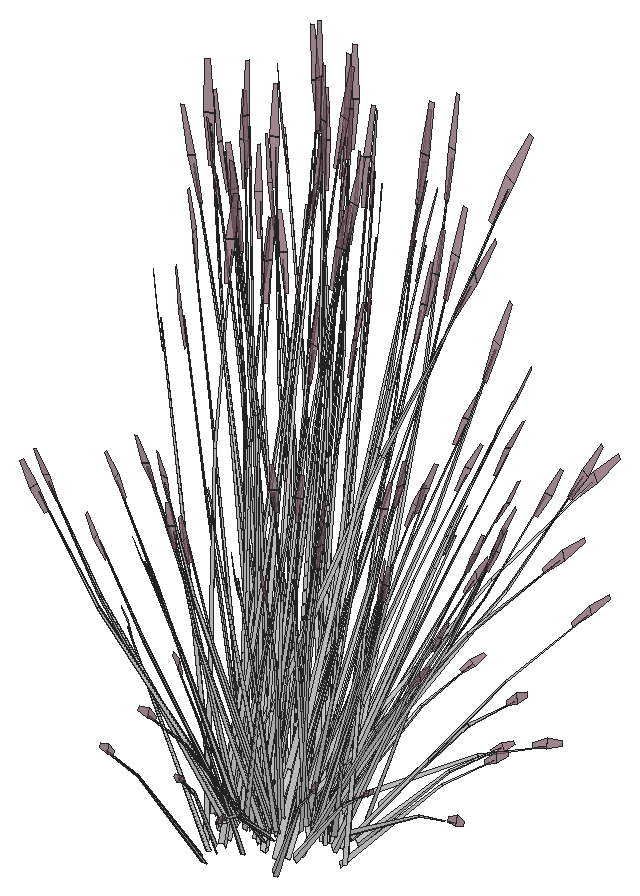
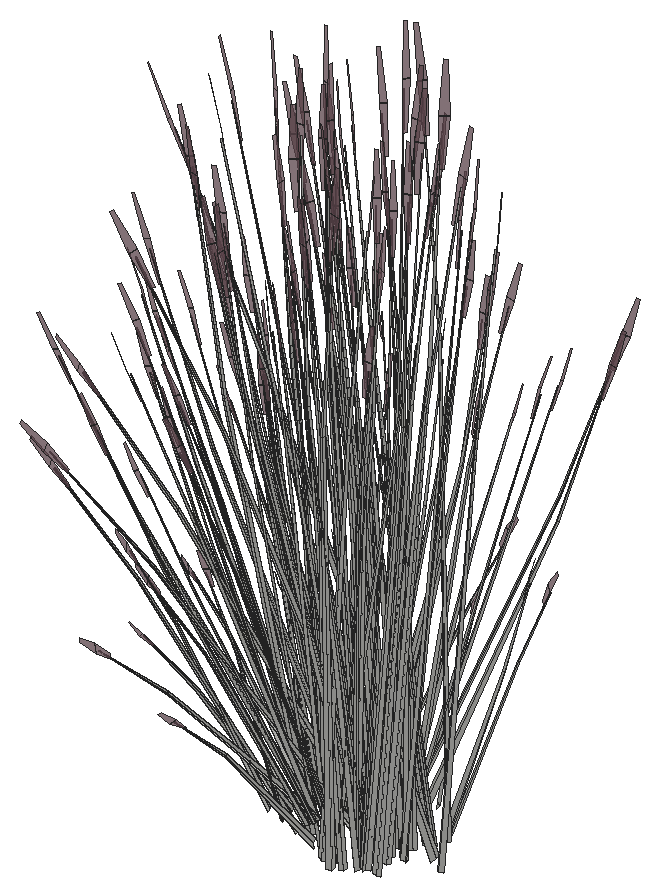
# SketchUp Ruby script. Lengths in inches.
U = 1.inch
M = Sketchup.active_model
def pt(a) = Geom::Point3d.new(a.map { |v| v * U })
def face(e, loops, mat)
  f = e.add_face(loops[0].map { |a| pt(a) })
  loops[1..].each { |l| e.add_face(l.map { |a| pt(a) }).erase! }
  f.material = f.back_material = mat if mat
  f
end
# faces: each face lists its corners as indices into pts; further lists are holes
def faces(e, pts, list, mat = nil) = list.each { |f| face(e, (f[0].is_a?(Array) ? f : [f]).map { |l| l.map { |i| pts[i] } }, mat) }
# xy, xz, yz: faces in a plane at the given z, y or x. An outline is a flat list of corners, or four numbers for a rectangle; further outlines are holes
def ring(l) = l.size == 4 ? [[l[0], l[1]], [l[2], l[1]], [l[2], l[3]], [l[0], l[3]]] : l.each_slice(2).to_a
def flat(e, list, mat, &to3) = list.each { |f| face(e, (f[0].is_a?(Array) ? f : [f]).map { |l| ring(l).map { |u, v| to3.(u, v) } }, mat) }
def xy(e, z, list, mat = nil) = flat(e, list, mat) { |x, y| [x, y, z] }
def xz(e, y, list, mat = nil) = flat(e, list, mat) { |x, z| [x, y, z] }
def yz(e, x, list, mat = nil) = flat(e, list, mat) { |y, z| [x, y, z] }
def lines(e, pts, list) = list.each { |a, b| e.add_line(pt(pts[a]), pt(pts[b])) }
# prism: a flat outline (further loops are holes) pulled along v
def prism(e, loops, v, mat = nil)
  f = face(e, loops, mat); d = Geom::Vector3d.new(v.map { |x| x * U })
  f.pushpull(f.normal.samedirection?(d) ? d.length : -d.length)
end
def box(e, o, s, mat = nil) = prism(e, [[o, [o[0] + s[0], o[1], o[2]], [o[0] + s[0], o[1] + s[1], o[2]], [o[0], o[1] + s[1], o[2]]]], [0, 0, s[2]], mat)
def at(x, y, z, deg = 0) = Geom::Transformation.translation(pt([x, y, z])) * Geom::Transformation.rotation(ORIGIN, Z_AXIS, deg.degrees)
def axes(o, x, y, z) = Geom::Transformation.new([*x, 0, *y, 0, *z, 0, *pt(o).to_a, 1])
def part(name) = M.definitions.add(name)
# library, detail: a bought-in or finely detailed component or shape, given as its bounding box
def library(name, o, s) = part(name).tap { |d| box(d.entities, o, s) }
def detail(e, o, s) = box(e.add_group.entities, o, s)
def put(e, d, t, mat = nil) = e.add_instance(d, t).tap { |i| i.material = mat if mat }
def group(e, t, mat = nil) = e.add_group.tap { |g| g.transformation = t; g.material = mat if mat }.entities
root = M.entities
M.materials.add("LightPink_Translucent").color = [144, 107, 117]
M.materials["LightPink_Translucent"].alpha = 0.75
c1 = part("blade")
p = [[2.15,0.21,22],[0,0.17,0],[0.09,0.45,0],[2.18,0.31,22],[2.29,0.31,22],[0.38,0.45,0],
  [2.48,0.24,33],[2.49,0.24,33],[2.48,0.22,33]]
faces(c1.entities,p,[[0,1,2,3],[4,5,2,3],[6,3,4,7],[8,0,3,6]])
c2 = part("seeds")
p = [[0.3,-0.1,1.38],[-0.01,-0.03,1.59],[-0.01,-0.03,0.03],[0.14,-0.07,-0.07],[0.29,-0.03,3],[0.15,0.01,3.11]]
faces(c2.entities,p,[[0,1,2,3],[1,0,4,5]],"LightPink_Translucent")
c3 = part("blade with seeds")
put(c3.entities,c1,at(0,0,0))
put(c3.entities,c2,axes([2.4,0.25,30.99],[1.5799,-0.05474,1.17369],[-0.12525,1.92788,0.29478],[-0.07173,-0.02425,1.56792]))
put(root,c3,axes([266.18,258.16,16.92],[-1.20468,-0.25962,-0.51099],[0.41292,-0.89013,-0.3958],[-0.11046,-0.35838,0.97773]))
put(root,c3,axes([261.53,261.37,14.26],[0.85545,-0.64616,-0.30978],[0.85545,0.64616,0.30978],[0,-0.20813,1.38974]))
put(root,c3,axes([265.39,257.19,14.36],[-0.84686,0.59414,-0.03893],[-0.77596,-0.65071,-0.17649],[-0.05463,-0.18438,0.58215]))
put(root,c3,axes([265.05,263.05,14.6],[1.54892,0.2182,0.45755],[-0.31522,1.23236,0.17955],[-0.22636,-0.119,1.58856]))
put(root,c3,axes([264.65,262.83,14.95],[-0.59459,0.93321,0.44739],[-1.23546,-0.44912,-0.21531],[0,-0.21512,1.43643]))
put(root,c3,axes([266.61,258.33,17.22],[-0.5849,-0.8421,-0.71045],[1.20401,-0.4693,0.08574],[-0.13677,-0.40688,1.00501]))
put(root,c3,axes([264.22,265.02,14.71],[1.31687,-0.27488,0.17642],[0.32517,1.02297,0.35086],[-0.11745,-0.14905,1.60407]))
put(root,c3,axes([265.92,265.18,14.43],[-1.23546,-0.46496,0],[0.59459,-0.96613,0],[0,0,1.62707]))
put(root,c3,axes([266.84,258.46,17.29],[-0.36946,0.79643,0.35414],[-1.07787,-0.23229,-0.4572],[-0.09883,-0.32066,0.87481]))
put(root,c3,axes([268.14,265.08,14.71],[0.35402,-1.02926,0.17642],[1.29548,0.29127,0.35086],[-0.22379,0.00501,1.60407]))
put(root,c3,axes([267.54,263.71,14.85],[0.90538,0.62224,0.1448],[-0.75521,0.70202,-0.41347],[-0.21021,0.09491,1.26744]))
put(root,c3,axes([267.22,262.94,14.53],[-1.1399,-0.8914,-0.06131],[1.1406,-0.89194,0],[-0.03981,-0.03113,1.75571]))
put(root,c3,axes([267.52,263.26,14.95],[1.33077,-0.06393,0.44739],[0.12035,1.06125,-0.21531],[-0.23824,0.10756,1.43643]))
put(root,c3,axes([267.84,265.7,14.57],[1.53422,0.33662,0.30756],[-0.38383,1.20322,-0.36492],[-0.25393,0.15059,1.64885]))
put(root,c3,axes([265.61,256.47,13.73],[-0.20555,0.03731,1.76342],[-1.13672,-0.42002,-0.26939],[0.01907,-0.35034,0.30037]))
put(root,c3,axes([268.5,265.63,14.71],[1.14694,-0.51783,0.49651],[0.68554,0.92854,0],[-0.26122,0.11794,1.57504]))
put(root,c3,axes([266.72,257.62,16.76],[0.36946,-0.79643,-0.35414],[1.07787,0.23229,0.4572],[-0.09883,-0.32066,0.87481]))
put(root,c3,axes([264.92,261.92,14.6],[0.53281,1.15808,0.45755],[-1.52239,0.4027,0.17955],[0.01861,-0.2128,1.58856]))
put(root,c3,axes([264.67,261.77,14.45],[0.59459,-0.93321,-0.44739],[1.23546,0.44912,0.21531],[0,-0.21512,1.43643]))
put(root,c3,axes([266.2,264.78,14.44],[-0.39985,-0.89288,0],[1.1418,-0.31268,0],[0,0,1.54371]))
put(root,c3,axes([267.8125,263.02,14.45],[-0.59459,0.93321,-0.44739],[-1.23546,-0.44912,0.21531],[0,0.21512,1.43643]))
put(root,c3,axes([267.18,257.74,16.97],[0.90301,-0.35198,0.0643],[0.44199,0.64184,0.50621],[-0.08721,-0.28293,0.77189]))
put(root,c3,axes([270.16,262.45,14.71],[-0.96285,-0.75439,0.17642],[0.97031,-0.7317,0.35086],[-0.10634,0.15406,1.60407]))
put(root,c3,axes([266.84,262.02,14.44],[0,-1.19833,0],[1.53239,0,0],[0,0,1.79456]))
put(root,c3,axes([266.86,257.8,16.97],[1.20755,0.27075,0.48003],[-0.41292,0.89013,0.3958],[-0.07257,-0.35005,0.9933]))
put(root,c3,axes([265.41,262.23,14.67],[1.3808,0.50196,0.24065],[-0.66454,1.04299,0.50002],[0,-0.24043,1.60543]))
put(root,c3,axes([267.61,262.49,14.53],[0,1.19774,-0.05637],[-1.53239,0,0],[0,0.03764,1.79368]))
put(root,c3,axes([264.97,261.54,14.95],[-1.33077,0.06393,0.44739],[-0.12035,-1.06125,-0.21531],[0.23824,-0.10756,1.43643]))
put(root,c3,axes([264.35,259.71,14.71],[-0.35402,1.02926,0.17642],[-1.29548,-0.29127,0.35086],[0.22379,-0.00501,1.60407]))
put(root,c3,axes([266.875,264.8125,14.53],[0.53281,1.18979,-0.06012],[-1.52239,0.41691,0],[0.01861,0.04155,1.72173]))
put(root,c3,axes([263.71,258.44,14.61],[-0.7662,-1.03778,0],[1.28187,-0.57875,-0.51607],[0.29196,-0.13181,1.63711]))
put(root,c3,axes([271.27,263.25,14.4375],[-1.53164,-0.00828,-0.04976],[0,-1.1575,0.49943],[-0.04813,0.2635,1.58352]))
put(root,c3,axes([268.26,259.77,14.71],[-1.31687,0.27488,0.17642],[-0.32517,-1.02297,0.35086],[0.11745,0.14905,1.60407]))
put(root,c3,axes([266.92,255.9375,15],[0.15721,0.60392,1.1486],[-0.87211,-0.33448,0.84392],[0.09385,-0.30923,0.25299]))
put(root,c3,axes([266.11,261.26,14.6],[-1.01611,0.93987,0.45755],[-1.20717,-0.82966,0.17955],[0.24496,-0.0938,1.58856]))
put(root,c3,axes([267.85,262.74,14.45],[0.85545,0.66896,0],[-0.85545,0.66896,0],[0,0,1.69266]))
put(root,c3,axes([267.83,261.96,14.95],[0.59459,-0.93321,0.44739],[1.23546,0.44912,-0.21531],[0,0.21512,1.43643]))
put(root,c3,axes([267.32,265.2,14.44],[1.23546,0.46496,0],[-0.59459,0.96613,0],[0,0,1.74954]))
put(root,c3,axes([267.43,261.74,14.62],[-1.54892,-0.2182,0.49198],[0.31522,-1.23236,0.19306],[0.22636,0.119,1.70813]))
put(root,c3,axes([270.65,256.92,16.95],[-0.12446,0.07911,1.77383],[-1.21937,-0.26689,-0.16761],[-0.04414,-0.34521,0.31391]))
put(root,c3,axes([269.7,259.21,17.27],[-1.34686,-0.05131,-0.1216],[0.03681,-0.97156,-0.67495],[0.09356,-0.37418,1.02557]))
put(root,c3,axes([270.95,263.42,14.26],[-0.85545,0.64616,-0.30978],[-0.85545,-0.64616,0.30978],[0,0.20813,1.38974]))
put(root,c3,axes([267.875,262.28,14.44],[1.37109,0,0],[0,1.07219,0],[0,0,1.78407]))
put(root,c3,axes([269.17,259.35,17.29],[-0.82919,0.54528,0.35414],[-0.78493,-0.62262,-0.4572],[0.11943,-0.31634,0.87481]))
put(root,c3,axes([266.56,261.1,14.95],[-0.73619,-0.86927,0.44739],[1.11511,-0.61213,-0.21531],[0.23824,0.10756,1.43643]))
put(root,c3,axes([265.22,261.31,14.9],[-0.1428,-1.18174,-0.29095],[1.48733,-0.07145,-0.50002],[0.26191,-0.15741,1.59708]))
put(root,c3,axes([268.35,262.17,14.85],[1.1418,-0.30203,0.1448],[0.39985,0.86246,-0.41347],[0,0.18981,1.26744]))
put(root,c3,axes([268.78,258.84,16.92],[-0.87728,-0.69587,-0.51099],[0.92674,-0.60943,-0.3958],[0.13348,-0.35356,0.97773]))
put(root,c3,axes([267.96,262.24,14.9],[1.38012,0.49416,-0.29095],[-0.66454,1.04299,-0.50002],[0.04337,0.25608,1.59708]))
put(root,c3,axes([265.02,258.69,14.26],[1.14332,0.25625,-0.30978],[-0.28787,0.90242,0.30978],[0.23049,-0.10406,1.38974]))
put(root,c3,axes([268.2,257.6,14.83],[-0.34835,0.20963,1.43002],[-1.04325,-0.36691,-0.30754],[0.19338,-0.4563,0.61141]))
put(root,c3,axes([270.96,262.48,14.71],[0,-1.03566,0.49651],[1.37109,0,0],[0,0.23588,1.57504]))
put(root,c3,axes([271.54,263.44,14.25],[0,1.03566,-0.49651],[-1.37109,0,0],[0,0.23588,1.57504]))
put(root,c3,axes([264.75,258.28,14.25],[1.14694,-0.51783,-0.49651],[0.68554,0.92854,0],[0.26122,-0.11794,1.57504]))
put(root,c3,axes([267.05,260.86,14.85],[0.23642,-0.92427,0.1448],[1.15506,0.16044,-0.41347],[0.21021,0.09491,1.26744]))
put(root,c3,axes([268.69,259.25,14.71],[-1.14694,-0.51783,0.49651],[0.68554,-0.92854,0],[0.26122,0.11794,1.57504]))
put(root,c3,axes([269.05,259.16,17.22],[0.03189,-0.95798,-0.71045],[1.34277,0.06434,0.08574],[0.14171,-0.40585,1.00501]))
put(root,c3,axes([267.69,264.66,14.42],[1.2866,-0.3514,-0.19198],[0.45209,1.01223,0.00008],[0.14202,-0.03884,1.73897]))
put(root,c3,axes([267.48,266.01,17.29],[-0.18927,-0.83419,0.35414],[1.08199,-0.22027,-0.4572],[0.29062,0.23905,0.87481]))
put(root,c3,axes([267.72,261.65,14.45],[0.73619,0.86927,-0.44739],[-1.11511,0.61213,0.21531],[0.23824,0.10756,1.43643]))
put(root,c3,axes([268.2,261.21,16.71],[-1.05895,-0.53811,1.38283],[1.11816,-0.83781,0.59665],[0.34166,0.5049,1.33663]))
put(root,c3,axes([269.6,258.58,16.76],[0.82919,-0.54528,-0.35414],[0.78493,0.62262,0.4572],[0.11943,-0.31634,0.87481]))
put(root,c3,axes([269.92,258.86,16.97],[1.00708,0.04826,0.0643],[-0.02761,0.72867,0.50621],[0.10538,-0.27912,0.77189]))
put(root,c3,axes([269.8,265.59,15],[-0.69001,-0.29779,1.1486],[0.89096,-0.30257,0.84392],[0.24031,0.2563,0.25299]))
put(root,c3,axes([270.92,257.66,16.95],[-0.01183,-0.20612,1.74944],[-0.99913,-0.59572,-0.27667],[0.15447,-0.36112,0.14031]))
put(root,c3,axes([266.11,260.41,14.3],[0.82544,-0.77843,-0.62353],[1.0254,0.70586,-0.16365],[0.33076,-0.19418,1.37633]))
put(root,c3,axes([269.6,258.79,16.97],[0.87265,0.70663,0.48003],[-0.92674,0.60943,0.3958],[0.16097,-0.33153,0.9933]))
put(root,c3,axes([269.73,259.72,14.26],[0.28787,0.90242,-0.30978],[-1.14332,0.25625,0.30978],[0.23049,0.10406,1.38974]))
put(root,c3,axes([271.89,262.66,14.61],[1.53239,0,0],[0,1.1575,-0.51607],[0,0.26363,1.63711]))
put(root,c3,axes([266.93,261.16,14.9],[1.23732,-0.68758,-0.29095],[0.8228,0.97154,-0.50002],[0.30528,0.09867,1.59708]))
put(root,c3,axes([270.61,261.04,17.29],[-1.06674,0.14801,0.35414],[-0.28168,-0.84611,-0.4572],[0.30569,-0.22726,0.87481]))
put(root,c3,axes([267.54,258.67,16.11],[-0.22818,0.35597,1.71376],[-0.95725,-0.73667,0.13857],[0.43183,-0.45914,0.73262]))
put(root,c3,axes([263.81,260.54,13.83],[-1.20625,0.41464,1.28929],[-0.38394,-1.1897,0.50096],[0.74071,0.01979,1.46642]))
put(root,c3,axes([271.16,261.12,17.27],[-1.1336,-0.57106,-0.1216],[0.65308,-0.827,-0.67495],[0.32027,-0.28747,1.02557]))
put(root,c3,axes([269.35,258.71,14.61],[0.7662,-1.03778,0],[1.28187,0.57875,-0.51607],[0.29196,0.13181,1.63711]))
put(root,c3,axes([270.64,258.25,13.73],[-0.18342,-0.08159,1.76342],[-0.47115,-0.9115,-0.26939],[0.31784,-0.24736,0.30037]))
put(root,c3,axes([269.63,264.88,17.29],[-0.69728,-0.64842,0.35414],[0.79619,-0.61382,-0.4572],[0.40453,0.09339,0.87481]))
put(root,c3,axes([270.05,259.33,14.25],[1.14694,0.51783,-0.49651],[-0.68554,0.92854,0],[0.26122,0.11794,1.57504]))
put(root,c3,axes([270.26,265.47,16.97],[-0.06171,0.78753,0.0643],[-0.9318,-0.02159,0.50621],[0.35694,0.08241,0.77189]))
put(root,c3,axes([270.35,265.22,16.97],[-0.90362,0.68241,0.48003],[-0.77932,-0.72471,0.3958],[0.42395,0.12588,0.9933]))
put(root,c3,axes([270.6,260.44,16.92],[-0.31482,-0.94565,-0.51099],[1.19224,-0.16542,-0.3958],[0.34166,-0.254,0.97773]))
put(root,c3,axes([272.7,265.32,16.17],[-0.23455,-0.87059,-0.03492],[1.10861,-0.20015,-0.15832],[0.23151,0.05519,0.52218]))
put(root,c3,axes([270.78,263.0625,17.29],[-1.01846,-0.28891,0.35414],[0.29705,-0.84289,-0.4572],[0.41005,-0.07729,0.87481]))
put(root,c3,axes([268.38,261.3125,14.3],[1.27479,0.1698,-0.62353],[-0.26901,1.04736,-0.16365],[0.38043,0.12691,1.37633]))
put(root,c3,axes([273.81,261.93,14.5],[-0.75977,-0.66224,-0.06488],[0.83212,-0.6068,-0.29416],[0.23578,-0.04272,0.97024]))
put(root,c3,axes([272.0625,258.56,15],[-0.40819,0.5272,1.1486],[-0.35086,-0.70831,0.84392],[0.33713,-0.17749,0.25299]))
put(root,c3,axes([271.58,260.91,16.97],[0.8413,0.43556,0.0643],[-0.48981,0.62025,0.50621],[0.26973,-0.20053,0.77189]))
put(root,c3,axes([271.34,260.72,16.97],[0.30393,0.95317,0.48003],[-1.19224,0.16542,0.3958],[0.35138,-0.22417,0.9933]))
put(root,c3,axes([268.12,263.56,16.11],[-0.45521,-0.17844,1.71376],[0.94204,-0.74856,0.13857],[0.58713,0.33769,0.73262]))
put(root,c3,axes([273.95,260.87,16.95],[-0.16006,-0.00787,1.77383],[-0.66468,-0.8428,-0.16761],[0.26693,-0.27711,0.31391]))
put(root,c3,axes([271.48,260.54,16.76],[1.06674,-0.14801,-0.35414],[0.28168,0.84611,0.4572],[0.30569,-0.22726,0.87481]))
put(root,c3,axes([270.63,260.82,17.22],[0.64013,-0.81717,-0.71045],[1.12174,0.58074,0.08574],[0.38221,-0.29607,1.00501]))
put(root,c3,axes([271.7,263.33,16.97],[0.4501,0.70615,0.0643],[-0.82077,0.34564,0.50621],[0.36181,-0.0682,0.77189]))
put(root,c3,axes([270.62,265.22,16.76],[0.69728,0.64842,-0.35414],[-0.79619,0.61382,0.4572],[0.40453,0.09339,0.87481]))
put(root,c3,axes([269.82,265.29,17.27],[0.06562,-1.05324,-0.1216],[1.2424,0.02879,-0.67495],[0.4785,0.07316,1.02557]))
put(root,c3,axes([271.21,263.35,17.27],[-0.6166,-0.93779,-0.1216],[1.09436,-0.46085,-0.67495],[0.46117,-0.12373,1.02557]))
put(root,c3,axes([271.62,263.07,16.97],[-0.34623,0.9443,0.48003],[-1.13828,-0.3229,0.3958],[0.44763,-0.05675,0.9933]))
put(root,c3,axes([270.9,264.66,16.95],[0.26289,-0.01751,1.74944],[0.72108,-0.8046,-0.27667],[0.46761,0.10621,0.14031]))
put(root,c3,axes([271.15,262.54,16.92],[0.332,-0.94205,-0.51099],[1.13828,0.3229,-0.3958],[0.45829,-0.08638,0.97773]))
put(root,c3,axes([274.01,263.14,15],[-0.75718,0.17097,1.1486],[0.35641,-0.70661,0.84392],[0.40168,0.04835,0.25299]))
put(root,c3,axes([271.56,260.07,14.83],[-0.4378,-0.03068,1.43002],[-0.44851,-0.8229,-0.30754],[0.53783,-0.23279,0.61141]))
put(root,c3,axes([271.85,262.97,16.76],[1.01846,0.28891,-0.35414],[-0.29705,0.84289,0.4572],[0.41005,-0.07729,0.87481]))
put(root,c3,axes([269.88,264.79,17.22],[1.22504,0.02494,-0.71045],[-0.08228,1.05005,0.08574],[0.51899,0.11081,1.00501]))
put(root,c3,axes([272.37,262.81,14.22],[-0.7893,0.12429,1.41583],[-0.12563,-0.9893,0.08104],[0.55282,-0.14974,0.80566]))
put(root,c3,axes([273.23,262.16,13.73],[-0.06405,-0.15723,1.76342],[0.44421,-0.91974,-0.26939],[0.4481,-0.01323,0.30037]))
put(root,c3,axes([273.66,266.13,16.95],[-0.11081,-0.09067,1.77383],[0.2424,-0.97188,-0.16761],[0.43649,-0.06209,0.31391]))
put(root,c3,axes([269.08,261.93,16.11],[-0.50831,0.02346,1.71376],[0.33721,-1.01661,0.13857],[0.72439,0.06288,0.73262]))
put(root,c3,axes([270.9375,262.88,17.22],[1.07686,-0.45739,-0.71045],[0.60013,0.94154,0.08574],[0.52031,-0.10696,1.00501]))
put(root,c3,axes([274.56,261.875,16.95],[0.17006,-0.15775,1.74944],[-0.21766,-0.96766,-0.27667],[0.42669,-0.18347,0.14031]))
put(root,c3,axes([272.59,264.28,14.83],[-0.29514,-0.25472,1.43002],[0.38401,-0.84262,-0.30754],[0.59714,0.11414,0.61141]))
